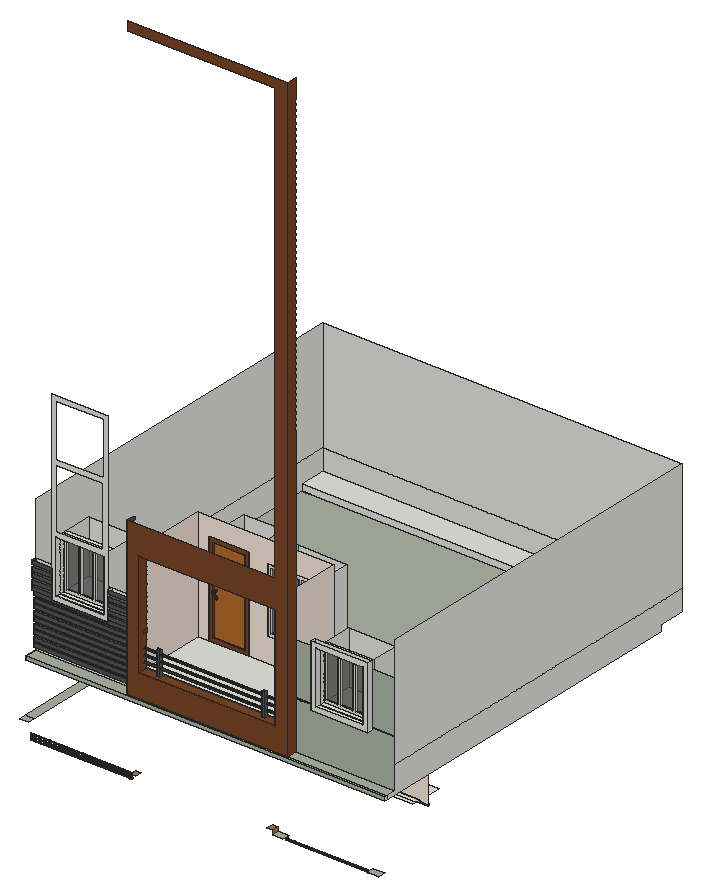
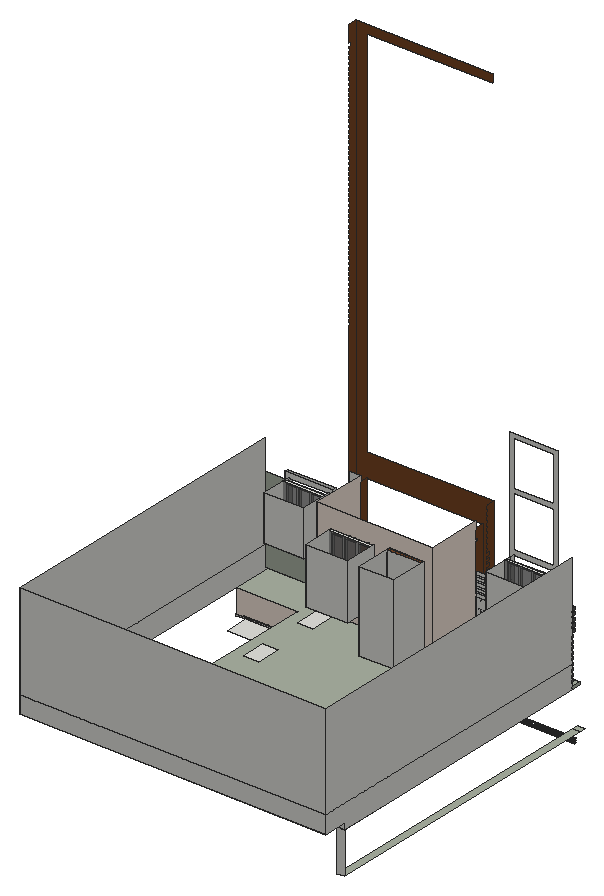
# SketchUp Ruby script. Lengths in inches.
U = 1.inch
M = Sketchup.active_model
def pt(a) = Geom::Point3d.new(a.map { |v| v * U })
def face(e, loops, mat)
  f = e.add_face(loops[0].map { |a| pt(a) })
  loops[1..].each { |l| e.add_face(l.map { |a| pt(a) }).erase! }
  f.material = f.back_material = mat if mat
  f
end
# faces: each face lists its corners as indices into pts; further lists are holes
def faces(e, pts, list, mat = nil) = list.each { |f| face(e, (f[0].is_a?(Array) ? f : [f]).map { |l| l.map { |i| pts[i] } }, mat) }
# xy, xz, yz: faces in a plane at the given z, y or x. An outline is a flat list of corners, or four numbers for a rectangle; further outlines are holes
def ring(l) = l.size == 4 ? [[l[0], l[1]], [l[2], l[1]], [l[2], l[3]], [l[0], l[3]]] : l.each_slice(2).to_a
def flat(e, list, mat, &to3) = list.each { |f| face(e, (f[0].is_a?(Array) ? f : [f]).map { |l| ring(l).map { |u, v| to3.(u, v) } }, mat) }
def xy(e, z, list, mat = nil) = flat(e, list, mat) { |x, y| [x, y, z] }
def xz(e, y, list, mat = nil) = flat(e, list, mat) { |x, z| [x, y, z] }
def yz(e, x, list, mat = nil) = flat(e, list, mat) { |y, z| [x, y, z] }
def lines(e, pts, list) = list.each { |a, b| e.add_line(pt(pts[a]), pt(pts[b])) }
# prism: a flat outline (further loops are holes) pulled along v
def prism(e, loops, v, mat = nil)
  f = face(e, loops, mat); d = Geom::Vector3d.new(v.map { |x| x * U })
  f.pushpull(f.normal.samedirection?(d) ? d.length : -d.length)
end
def box(e, o, s, mat = nil) = prism(e, [[o, [o[0] + s[0], o[1], o[2]], [o[0] + s[0], o[1] + s[1], o[2]], [o[0], o[1] + s[1], o[2]]]], [0, 0, s[2]], mat)
def at(x, y, z, deg = 0) = Geom::Transformation.translation(pt([x, y, z])) * Geom::Transformation.rotation(ORIGIN, Z_AXIS, deg.degrees)
def axes(o, x, y, z) = Geom::Transformation.new([*x, 0, *y, 0, *z, 0, *pt(o).to_a, 1])
def part(name) = M.definitions.add(name)
# library, detail: a bought-in or finely detailed component or shape, given as its bounding box
def library(name, o, s) = part(name).tap { |d| box(d.entities, o, s) }
def detail(e, o, s) = box(e.add_group.entities, o, s)
def put(e, d, t, mat = nil) = e.add_instance(d, t).tap { |i| i.material = mat if mat }
def group(e, t, mat = nil) = e.add_group.tap { |g| g.transformation = t; g.material = mat if mat }.entities
root = M.entities
M.materials.add("Generic\#1").color = [85, 85, 85]
M.materials.add("Generic\#2").color = [170, 178, 163]
M.materials.add("Generic\#3").color = [162, 123, 74]
M.materials.add("Generic\#4").color = [241, 227, 216]
M.materials.add("[Color M07]").color = [58, 58, 58]
M.materials.add("[Translucent Glass Gray]").color = [91, 91, 91]
M.materials["[Translucent Glass Gray]"].alpha = 0.55
M.materials.add("[Wood Bamboo]").color = [177, 105, 43]
M.materials.add("[Wood Veneer 01]").color = [120, 70, 37]
c1 = part("Group\#4")
xy(c1.entities,0,[[0,0,168,3.625]])
xy(c1.entities,5.375,[[0,0,168,3.625]])
xz(c1.entities,0,[[0,0,168,5.375]])
yz(c1.entities,0,[[0,0,3.625,5.375]])
c2 = part("Group\#3")
xy(c2.entities,0,[[0,4.93,60.125,10.18]])
xy(c2.entities,5.66,[[5.66,4.93,54.46,7.18]],"[Wood Veneer 01]")
xy(c2.entities,68.44,[[8.18,1.47,8.18,7.18,9.93,7.18,9.93,2.62]],"[Color M07]")
xy(c2.entities,70.41,[[8.19,0,9.94,1.15,9.94,7.18,8.19,7.18]],"[Color M07]")
xy(c2.entities,134.78,[[5.66,4.93,54.46,7.18]])
xy(c2.entities,140.4375,[[0,4.93,60.125,10.18]],"[Wood Veneer 01]")
xz(c2.entities,4.93,[[[0,0,60.125,140.4375],[5.66,5.66,54.46,134.78]]],"[Wood Veneer 01]")
xz(c2.entities,7.18,[[[5.66,5.66,54.46,134.78],[8.18,68.44,8.19,70.41,9.94,70.41,9.93,68.44]],[8.18,68.44,8.19,70.41,9.94,70.41,9.93,68.44]],"[Wood Bamboo]")
xz(c2.entities,10.18,[[0,0,60.125,140.4375]])
yz(c2.entities,0,[[4.93,0,10.18,140.4375]],"[Wood Veneer 01]")
yz(c2.entities,5.66,[[4.93,5.66,7.18,134.78]],"[Wood Veneer 01]")
yz(c2.entities,54.46,[[4.93,5.66,7.18,134.78]],"[Wood Veneer 01]")
yz(c2.entities,60.125,[[4.93,0,10.18,140.4375]],"[Wood Veneer 01]")
p = [[8.19,0,70.41],[8.18,1.47,68.44],[14.45,1.47,61.21],[15.43,0,62.06],[15.45,2.62,62.07],[16.43,1.15,62.92],
  [9.93,2.62,68.44],[9.94,1.15,70.41],[8.19,7.18,70.41],[8.18,7.18,68.44],[9.93,7.18,68.44],[9.94,7.18,70.41],
  [8.95,0.93,69.83],[15.58,0.93,62.1875],[8.95,7.18,69.83]]
faces(c2.entities,p,[[0,1,2,3],[3,2,4,5],[1,6,4,2],[7,0,3,5],[6,7,5,4],[8,9,1,0],[10,11,7,6]],"[Color M07]")
lines(c2.entities,p,[[12,13],[14,12]])
c3 = part("Group\#2")
xy(c3.entities,0,[[0,0,74.5625,5.5]])
xy(c3.entities,4.83,[[4.83,0,23.24,2.5],[28.07,0,46.49,2.5],[51.32,0,69.73,2.5]])
xy(c3.entities,93.17,[[4.83,0,23.24,2.5],[28.07,0,46.49,2.5],[51.32,0,69.73,2.5]])
xy(c3.entities,98,[[0,0,74.5625,5.5]])
xz(c3.entities,0,[[[0,0,74.5625,98],[28.07,4.83,46.49,93.17],[51.32,4.83,69.73,93.17],[4.83,4.83,23.24,93.17]]])
xz(c3.entities,2.5,[[4.83,4.83,23.24,93.17],[28.07,4.83,46.49,93.17],[51.32,4.83,69.73,93.17]],"[Translucent Glass Gray]")
xz(c3.entities,5.5,[[0,0,74.5625,98]],"[Translucent Glass Gray]")
yz(c3.entities,0,[[0,0,5.5,98]])
yz(c3.entities,4.83,[[0,4.83,2.5,93.17]])
yz(c3.entities,23.24,[[0,4.83,2.5,93.17]])
yz(c3.entities,28.07,[[0,4.83,2.5,93.17]])
yz(c3.entities,46.49,[[0,4.83,2.5,93.17]])
yz(c3.entities,51.32,[[0,4.83,2.5,93.17]])
yz(c3.entities,69.73,[[0,4.83,2.5,93.17]])
yz(c3.entities,74.5625,[[0,0,5.5,98]])
c4 = part("Group\#1")
xy(c4.entities,0,[[0,0,70.8125,6.0625]])
xy(c4.entities,4.26,[[4.26,0,22.19,2.0625],[26.44,0,44.37,2.0625],[48.63,0,66.56,2.0625]])
xy(c4.entities,75.06,[[4.26,0,22.19,2.0625],[26.44,0,44.37,2.0625],[48.63,0,66.56,2.0625]])
xy(c4.entities,79.3125,[[0,0,70.8125,6.0625]])
xz(c4.entities,0,[[[0,0,70.8125,79.3125],[26.44,4.26,44.37,75.06],[4.26,4.26,22.19,75.06],[48.63,4.26,66.56,75.06]]])
xz(c4.entities,2.0625,[[4.26,4.26,22.19,75.06],[26.44,4.26,44.37,75.06],[48.63,4.26,66.56,75.06]],"[Translucent Glass Gray]")
xz(c4.entities,6.0625,[[0,0,70.8125,79.3125]],"[Translucent Glass Gray]")
yz(c4.entities,0,[[0,0,6.0625,79.3125]])
yz(c4.entities,4.26,[[0,4.26,2.0625,75.06]])
yz(c4.entities,22.19,[[0,4.26,2.0625,75.06]])
yz(c4.entities,26.44,[[0,4.26,2.0625,75.06]])
yz(c4.entities,44.37,[[0,4.26,2.0625,75.06]])
yz(c4.entities,48.63,[[0,4.26,2.0625,75.06]])
yz(c4.entities,66.56,[[0,4.26,2.0625,75.06]])
yz(c4.entities,70.8125,[[0,0,6.0625,79.3125]])
xy(root,58.9,[[16.75,5.31,169.3125,6.62]],"Generic\#1")
xy(root,59.38,[[410.9,5.97,412.55,5.97,412.7,6.16,412.8125,6.43,412.85,6.72,412.8125,7.02,412.7,7.29,412.55,7.48,410.9,7.48,410.75,7.29,410.64,7.02,410.6,6.72,410.64,6.43,410.75,6.16],[512.09,5.97,513.74,5.97,513.89,6.16,514,6.43,514.04,6.72,514,7.02,513.89,7.29,513.74,7.48,512.09,7.48,511.94,7.29,511.83,7.02,511.79,6.72,511.83,6.43,511.94,6.16]])
xy(root,59.38,[[411.73,5.6,412.02,5.64,412.29,5.75,412.52,5.93,412.55,5.97,410.9,5.97,410.93,5.93,411.17,5.75,411.4375,5.64],[512.92,5.6,513.21,5.64,513.48,5.75,513.71,5.93,513.74,5.97,512.09,5.97,512.12,5.93,512.35,5.75,512.625,5.64],[410.9,7.48,412.55,7.48,412.52,7.52,412.29,7.7,412.02,7.8125,411.73,7.85,411.4375,7.8125,411.17,7.7,410.93,7.52],[512.09,7.48,513.74,7.48,513.71,7.52,513.48,7.7,513.21,7.8125,512.92,7.85,512.625,7.8125,512.35,7.7,512.12,7.52]],"Generic\#1")
xy(root,59.84,[[16.75,5.31,169.3125,6.62]],"Generic\#1")
xy(root,61.1875,[[383.68,1.625,399.68,12.1875],[526.51,1.625,543.6875,12.1875]],"Generic\#2")
xy(root,62.53,[[16.75,5.31,169.3125,6.62]],"Generic\#1")
xy(root,63.47,[[16.75,5.31,169.3125,6.62]],"Generic\#1")
xy(root,66.15,[[16.75,5.31,169.3125,6.62]],"Generic\#1")
xy(root,67.09,[[16.75,5.31,169.3125,6.62]],"Generic\#1")
xy(root,67.4375,[[43.38,5.24,44.57,6.49],[92.71,5.24,93.9,6.49],[142.04,5.24,143.23,6.49]],"Generic\#1")
xy(root,67.5625,[[169.3125,1.625,177.3125,12.1875],[375.68,1.625,383.68,12.1875]],"Generic\#3")
xy(root,84.25,[[3.6875,1.625,16.75,12.1875],[3.6875,12.1875,16.75,531.1875]],"Generic\#2")
xy(root,114.9375,[[455.38,87.75,526.46,94.125],[455.38,94.125,526.46,135.5]])
xy(root,115.46,[[435.75,94.125,451.03,95.75],[530.8125,94.125,543.6875,95.75]])
xy(root,117.46,[[435.75,94.125,451.03,95.75],[530.8125,94.125,543.6875,95.75]])
xy(root,119.29,[[451.03,87.75,530.8125,94.125]])
xy(root,158.4375,[[3.6875,12.1875,543.6875,15.8125],[3.6875,15.8125,3.6875,531.1875,435.75,531.1875,435.75,94.125,543.6875,94.125,543.6875,15.8125]],"Generic\#2")
xy(root,163.8125,[[153.3125,15.8125,395.4375,31.0625],[142.43,83.81,169.24,125.75],[383.68,83.81,410.49,125.75],[142.43,202,169.24,243.94],[383.68,202,410.49,243.94],
  [142.43,320.19,169.24,362.12],[383.68,320.19,410.49,320.19,410.49,362.12,383.68,362.12,383.68,361.87,405.71,361.87,405.71,322.81,383.68,322.81],[380.34,322.81,383.68,361.87],[383.68,322.81,405.71,361.87]])
xy(root,163.8125,[[3.6875,12.1875,543.6875,12.1875,543.6875,15.8125,153.3125,15.8125,153.3125,31.0625,3.6875,31.0625],[395.4375,15.8125,543.6875,31.0625]],"Generic\#2")
xy(root,168,[[3.6875,531.1875,543.6875,571.0625]])
xy(root,198.875,[[351.19,22.73,355.76,26.42],[171.6875,31.0625,171.6875,127,187.38,127,187.38,193.75,247.51,193.75,247.51,127,375.6875,127,375.6875,31.0625]])
xy(root,198.875,[[[171.6875,15.8125,375.6875,31.0625],[351.19,22.73,355.76,26.42],[192.01,22.73,196.57,26.42]]],"[Wood Veneer 01]")
xy(root,209.02,[[171.6875,23.99,375.6875,25.8]],"Generic\#1")
xy(root,210.64,[[171.6875,23.99,375.6875,25.8]],"Generic\#1")
xy(root,218.27,[[171.6875,23.99,375.6875,25.8]],"Generic\#1")
xy(root,219.89,[[171.6875,23.99,375.6875,25.8]],"Generic\#1")
xy(root,227.52,[[171.6875,23.99,375.6875,25.8]],"Generic\#1")
xy(root,229.14,[[171.6875,23.99,375.6875,25.8]],"Generic\#1")
xy(root,233.03,[[423.8125,24.0625,508.98,31.0625]])
xy(root,234.1875,[[192.01,22.73,196.57,26.42],[351.19,22.73,355.76,26.42]],"Generic\#1")
xy(root,235.875,[[395.4375,31.0625,423.8125,32.9375],[508.98,31.0625,543.6875,32.9375]])
xy(root,235.91,[[275.98,127,350.54,183.625]])
xy(root,237.875,[[395.4375,31.0625,423.8125,32.9375],[508.98,31.0625,543.6875,32.9375]])
xy(root,240.2,[[430.99,24.0625,501.8,31.0625],[430.99,31.0625,501.8,85.4375]])
xy(root,245.21,[[33.1875,24.0625,118.35,31.0625]],"Generic\#1")
xy(root,247.625,[[3.6875,24.0625,33.1875,31.0625],[118.35,24.0625,153.3125,31.0625]],"Generic\#1")
xy(root,252.39,[[40.36,24.0625,111.18,31.0625],[40.36,31.0625,111.18,85.4375]])
xy(root,253,[[3.6875,24.0625,33.1875,31.0625],[118.35,24.0625,153.3125,31.0625]],"Generic\#1")
xy(root,256.3125,[[3.6875,24.0625,33.1875,31.0625],[118.35,24.0625,153.3125,31.0625]],"Generic\#1")
xy(root,261.6875,[[3.6875,24.0625,33.1875,31.0625],[118.35,24.0625,153.3125,31.0625]],"Generic\#1")
xy(root,265,[[3.6875,24.0625,33.1875,31.0625],[118.35,24.0625,153.3125,31.0625]],"Generic\#1")
xy(root,270.375,[[3.6875,24.0625,33.1875,31.0625],[118.35,24.0625,153.3125,31.0625]],"Generic\#1")
xy(root,273.6875,[[3.6875,24.0625,33.1875,31.0625],[118.35,24.0625,153.3125,31.0625]],"Generic\#1")
xy(root,279.0625,[[118.35,31.0625,153.3125,35.3125]])
xy(root,279.0625,[[3.6875,24.0625,33.1875,31.0625],[118.35,24.0625,153.3125,31.0625]],"Generic\#1")
xy(root,282.375,[[118.35,31.0625,153.3125,35.3125]])
xy(root,282.375,[[3.6875,24.0625,33.1875,31.0625],[118.35,24.0625,153.3125,31.0625]],"Generic\#1")
xz(root,5.31,[[16.75,58.9,169.3125,59.84],[16.75,62.53,169.3125,63.47],[16.75,66.15,169.3125,67.09]],"Generic\#1")
xz(root,6.62,[[16.75,58.9,169.3125,59.84],[16.75,62.53,169.3125,63.47],[16.75,66.15,169.3125,67.09]])
xz(root,12.1875,[[3.6875,158.4375,543.6875,163.8125]],"Generic\#2")
xz(root,15.8125,[[[153.3125,163.8125,395.4375,163.8125,395.4375,1071.875,154.5,1071.875,154.5,1058.1875,375.6875,1058.1875,375.6875,397.75,153.3125,397.75],[171.6875,198.875,375.6875,356.125]]],"[Wood Veneer 01]")
xz(root,22.73,[[192.01,198.875,196.57,234.1875],[351.19,198.875,355.76,234.1875]],"Generic\#1")
xz(root,23.99,[[171.6875,209.02,375.6875,210.64],[171.6875,218.27,375.6875,219.89],[171.6875,227.52,375.6875,229.14]],"Generic\#1")
xz(root,24.0625,[[[423.8125,233.03,508.98,326.69],[430.99,240.2,501.8,319.52]],[[33.1875,245.21,118.35,522.69],[40.375,338.88,110.67,429.03],[40.36,252.39,111.18,331.7],[40.36,436.2,111.18,515.52]]])
xz(root,24.0625,[[3.6875,247.625,33.1875,253],[118.35,247.625,153.3125,253],[153.3125,247.625,171.6875,253],[40.36,252.39,111.18,253],[3.6875,256.3125,33.1875,261.6875],
  [118.35,256.3125,153.3125,261.6875],[3.6875,265,33.1875,270.375],[118.35,265,153.3125,270.375],[3.6875,273.6875,33.1875,279.0625],[118.35,273.6875,153.3125,279.0625],
  [3.6875,282.375,33.1875,287.75],[118.35,282.375,153.3125,287.75]],"Generic\#1")
xz(root,25.8,[[171.6875,209.02,375.6875,210.64],[171.6875,218.27,375.6875,219.89],[171.6875,227.52,375.6875,229.14]])
xz(root,26.42,[[192.01,198.875,196.57,234.1875],[351.19,198.875,355.76,234.1875]])
xz(root,31.0625,[[3.6875,163.8125,153.3125,163.8125,153.3125,247.625,118.35,247.625,118.35,245.21,33.1875,245.21,33.1875,247.625,3.6875,247.625],[153.3125,163.8125,395.4375,198.875],[153.3125,198.875,171.6875,247.625],[375.6875,198.875,395.4375,366.875],[[423.8125,233.03,508.98,326.69],[430.99,240.2,501.8,319.52]],
  [33.1875,245.21,118.35,247.625],[3.6875,247.625,33.1875,253],[33.1875,247.625,33.1875,253,40.36,253,40.36,252.39,111.18,252.39,111.18,253,118.35,253,118.35,247.625],[118.35,247.625,153.3125,253],[153.3125,247.625,171.6875,253],
  [3.6875,253,33.1875,256.3125],[33.1875,253,40.36,256.3125],[111.18,253,118.35,256.3125],[118.35,253,153.3125,256.3125],[153.3125,253,171.6875,256.3125],
  [3.6875,256.3125,33.1875,261.6875],[33.1875,256.3125,40.36,261.6875],[111.18,256.3125,118.35,261.6875],[118.35,256.3125,153.3125,261.6875],[153.3125,256.3125,171.6875,261.6875],
  [3.6875,261.6875,33.1875,265],[33.1875,261.6875,40.36,265],[111.18,261.6875,118.35,265],[118.35,261.6875,153.3125,265],[153.3125,261.6875,171.6875,265],
  [3.6875,265,33.1875,270.375],[33.1875,265,40.36,270.375],[111.18,265,118.35,270.375],[118.35,265,153.3125,270.375],[153.3125,265,171.6875,270.375],
  [3.6875,270.375,33.1875,273.6875],[33.1875,270.375,40.36,273.6875],[111.18,270.375,118.35,273.6875],[118.35,270.375,153.3125,273.6875],[153.3125,270.375,171.6875,273.6875],
  [3.6875,273.6875,33.1875,279.0625],[33.1875,273.6875,40.36,279.0625],[111.18,273.6875,118.35,279.0625],[118.35,273.6875,153.3125,279.0625],[153.3125,273.6875,171.6875,279.0625],
  [3.6875,279.0625,33.1875,282.375],[33.1875,279.0625,40.36,282.375],[111.18,279.0625,118.35,282.375],[118.35,279.0625,153.3125,282.375],[153.3125,279.0625,171.6875,282.375],
  [3.6875,282.375,33.1875,287.75],[33.1875,282.375,40.36,287.75],[111.18,282.375,118.35,287.75],[118.35,282.375,153.3125,287.75],[153.3125,282.375,171.6875,287.75]])
xz(root,31.0625,[[395.4375,163.8125,543.6875,163.8125,543.6875,235.875,508.98,235.875,508.98,233.03,423.8125,233.03,423.8125,235.875,395.4375,235.875],[395.4375,237.875,423.8125,315.5],[508.98,237.875,543.6875,315.5]],"Generic\#2")
xz(root,32.9375,[[395.4375,235.875,423.8125,237.875],[508.98,235.875,543.6875,237.875]],"Generic\#1")
xz(root,35.3125,[[118.35,279.0625,153.3125,282.375]])
xz(root,85.4375,[[430.99,240.2,501.8,319.52],[40.36,252.39,111.18,331.7]])
xz(root,94.125,[[451.03,115.46,530.8125,117.46],[451.03,117.46,530.8125,119.29]])
xz(root,94.125,[[435.75,117.46,451.03,117.46,451.03,119.29,530.8125,119.29,530.8125,117.46,543.6875,117.46,543.6875,158.4375,435.75,158.4375]],"Generic\#4")
xz(root,95.75,[[435.75,115.46,451.03,117.46],[530.8125,115.46,543.6875,117.46]])
xz(root,127,[[[171.6875,198.875,187.38,198.875,187.38,339.3125,247.51,339.3125,247.51,198.875,375.6875,198.875,375.6875,366.875,171.6875,366.875],[275.98,235.91,350.54,333.91]]],"Generic\#4")
xz(root,183.625,[[275.98,235.91,350.54,333.91]])
xz(root,193.75,[[187.38,198.875,247.51,339.3125]])
xz(root,531.1875,[[3.6875,84.25,16.75,158.4375],[3.6875,158.4375,543.6875,168]])
xz(root,571.0625,[[3.6875,168,543.6875,198.875],[3.6875,198.875,543.6875,366.875]])
yz(root,3.6875,[[31.0625,158.4375,31.0625,198.875,571.0625,198.875,571.0625,168,531.1875,168,531.1875,158.4375],[31.0625,198.875,571.0625,366.875]])
yz(root,3.6875,[[24.0625,247.625,31.0625,253],[24.0625,256.3125,31.0625,261.6875],[24.0625,265,31.0625,270.375],[24.0625,273.6875,31.0625,279.0625],[24.0625,282.375,31.0625,287.75]],"Generic\#1")
yz(root,3.6875,[[12.1875,158.4375,31.0625,163.8125]],"Generic\#2")
yz(root,16.75,[[5.31,58.9,6.62,59.84],[5.31,62.53,6.62,63.47],[5.31,66.15,6.62,67.09]],"Generic\#2")
yz(root,33.1875,[[24.0625,245.21,31.0625,247.625],[24.0625,247.625,31.0625,253],[24.0625,253,31.0625,256.3125],[24.0625,256.3125,31.0625,261.6875],[24.0625,261.6875,31.0625,265],
  [24.0625,265,31.0625,270.375],[24.0625,270.375,31.0625,273.6875],[24.0625,273.6875,31.0625,279.0625],[24.0625,279.0625,31.0625,282.375],[24.0625,282.375,31.0625,287.75]])
yz(root,40.36,[[24.0625,252.39,31.0625,331.7],[31.0625,252.39,85.4375,331.7]])
yz(root,111.18,[[24.0625,252.39,31.0625,331.7],[31.0625,252.39,85.4375,331.7]])
yz(root,118.35,[[24.0625,245.21,31.0625,247.625],[24.0625,247.625,31.0625,253],[24.0625,253,31.0625,256.3125],[24.0625,256.3125,31.0625,261.6875],[24.0625,261.6875,31.0625,265],
  [24.0625,265,31.0625,270.375],[24.0625,270.375,31.0625,273.6875],[24.0625,273.6875,31.0625,279.0625],[24.0625,279.0625,31.0625,282.375],[31.0625,279.0625,35.3125,282.375],
  [24.0625,282.375,31.0625,287.75]])
yz(root,153.3125,[[24.0625,247.625,31.0625,253],[24.0625,256.3125,31.0625,261.6875],[24.0625,265,31.0625,270.375],[24.0625,273.6875,31.0625,279.0625],[31.0625,279.0625,35.3125,282.375],
  [24.0625,282.375,31.0625,287.75]])
yz(root,153.3125,[[15.8125,163.8125,15.8125,397.75,27.4375,397.75,27.4375,395.3125,31.0625,395.3125,31.0625,392,27.4375,392,27.4375,386.625,31.0625,386.625,31.0625,383.3125,27.4375,383.3125,27.4375,377.9375,31.0625,377.9375,31.0625,374.625,27.4375,374.625,27.4375,369.25,31.0625,369.25,31.0625,365.9375,27.4375,365.9375,27.4375,360.5625,31.0625,360.5625,31.0625,357.25,27.4375,357.25,27.4375,351.875,31.0625,351.875,31.0625,348.5625,27.4375,348.5625,27.4375,343.1875,31.0625,343.1875,31.0625,338.88,27.75,338.88,27.75,334.5,31.0625,334.5,31.0625,331.1875,27.75,331.1875,27.75,325.8125,31.0625,325.8125,31.0625,322.5,24.0625,322.5,24.0625,317.125,31.0625,317.125,31.0625,313.8125,24.0625,313.8125,24.0625,308.4375,31.0625,308.4375,31.0625,305.125,24.0625,305.125,24.0625,299.75,31.0625,299.75,31.0625,296.4375,24.0625,296.4375,24.0625,291.0625,31.0625,291.0625,31.0625,287.75,24.0625,287.75,24.0625,282.375,31.0625,282.375,31.0625,279.0625,24.0625,279.0625,24.0625,273.6875,31.0625,273.6875,31.0625,270.375,24.0625,270.375,24.0625,265,31.0625,265,31.0625,261.6875,24.0625,261.6875,24.0625,256.3125,31.0625,256.3125,31.0625,253,24.0625,253,24.0625,247.625,31.0625,247.625,31.0625,163.8125]],"[Wood Veneer 01]")
yz(root,169.3125,[[5.31,58.9,6.62,59.84],[5.31,62.53,6.62,63.47],[5.31,66.15,6.62,67.09]])
yz(root,171.6875,[[23.99,209.02,25.8,210.64],[23.99,218.27,25.8,219.89],[23.99,227.52,25.8,229.14]])
yz(root,171.6875,[[31.0625,198.875,127,366.875]],"Generic\#4")
yz(root,171.6875,[[[15.8125,198.875,31.0625,198.875,31.0625,247.625,24.0625,247.625,24.0625,253,31.0625,253,31.0625,334.5,27.75,334.5,27.75,338.88,31.0625,338.88,31.0625,356.125,15.8125,356.125],[23.99,227.52,25.8,229.14],[23.99,218.27,25.8,219.89],[23.99,209.02,25.8,210.64]],[24.0625,247.625,31.0625,253]],"[Wood Veneer 01]")
yz(root,187.38,[[127,198.875,193.75,339.3125]])
yz(root,192.01,[[22.73,198.875,26.42,234.1875]],"Generic\#1")
yz(root,196.57,[[22.73,198.875,26.42,234.1875]],"Generic\#1")
yz(root,247.51,[[127,198.875,193.75,339.3125]])
yz(root,275.98,[[127,235.91,183.625,333.91]])
yz(root,350.54,[[127,235.91,183.625,333.91]])
yz(root,351.19,[[22.73,198.875,26.42,234.1875]],"Generic\#1")
yz(root,355.76,[[22.73,198.875,26.42,234.1875]],"Generic\#1")
yz(root,375.6875,[[31.0625,198.875,127,366.875]],"Generic\#4")
yz(root,375.6875,[[[15.8125,198.875,31.0625,356.125],[23.99,209.02,25.8,210.64],[23.99,218.27,25.8,219.89],[23.99,227.52,25.8,229.14]]],"[Wood Veneer 01]")
yz(root,383.68,[[1.625,61.1875,12.1875,67.5625]],"Generic\#3")
yz(root,395.4375,[[31.0625,235.875,32.9375,237.875]])
yz(root,395.4375,[[15.8125,163.8125,31.0625,163.8125,31.0625,596.625,28.5,596.625,28.5,602.125,31.0625,602.125,31.0625,604.9375,28.5,604.9375,28.5,610.4375,31.0625,610.4375,31.0625,613.25,28.5,613.25,28.5,618.75,31.0625,618.75,31.0625,621.5625,28.5,621.5625,28.5,627.0625,31.0625,627.0625,31.0625,629.875,28.5,629.875,28.5,635.375,31.0625,635.375,31.0625,638.1875,28.5,638.1875,28.5,643.6875,31.0625,643.6875,31.0625,646.5,28.5,646.5,28.5,652,31.0625,652,31.0625,654.8125,28.5,654.8125,28.5,660.3125,31.0625,660.3125,31.0625,663.125,28.5,663.125,28.5,668.625,31.0625,668.625,31.0625,671.4375,28.5,671.4375,28.5,676.9375,31.0625,676.9375,31.0625,679.75,28.5,679.75,28.5,685.25,31.0625,685.25,31.0625,688.0625,28.5,688.0625,28.5,693.5625,31.0625,693.5625,31.0625,696.375,28.5,696.375,28.5,701.875,31.0625,701.875,31.0625,704.6875,28.5,704.6875,28.5,710.1875,31.0625,710.1875,31.0625,713,28.5,713,28.5,718.5,31.0625,718.5,31.0625,721.3125,28.5,721.3125,28.5,726.8125,31.0625,726.8125,31.0625,729.625,28.5,729.625,28.5,735.125,31.0625,735.125,31.0625,737.9375,28.5,737.9375,28.5,743.4375,31.0625,743.4375,31.0625,746.25,28.5,746.25,28.5,751.75,31.0625,751.75,31.0625,754.5625,28.5,754.5625,28.5,760.0625,31.0625,760.0625,31.0625,762.875,28.5,762.875,28.5,768.375,31.0625,768.375,31.0625,771.1875,28.5,771.1875,28.5,776.6875,31.0625,776.6875,31.0625,779.5,28.5,779.5,28.5,785,31.0625,785,31.0625,787.8125,28.5,787.8125,28.5,793.3125,31.0625,793.3125,31.0625,796.125,28.5,796.125,28.5,801.625,31.0625,801.625,31.0625,804.4375,28.5,804.4375,28.5,809.9375,31.0625,809.9375,31.0625,812.75,28.5,812.75,28.5,818.25,31.0625,818.25,31.0625,821.0625,28.5,821.0625,28.5,826.5625,31.0625,826.5625,31.0625,829.375,28.5,829.375,28.5,834.875,31.0625,834.875,31.0625,837.6875,28.5,837.6875,28.5,843.1875,31.0625,843.1875,31.0625,846,28.5,846,28.5,851.5,31.0625,851.5,31.0625,854.3125,28.5,854.3125,28.5,859.8125,31.0625,859.8125,31.0625,862.625,28.5,862.625,28.5,868.125,31.0625,868.125,31.0625,870.9375,28.5,870.9375,28.5,876.4375,31.0625,876.4375,31.0625,879.25,28.5,879.25,28.5,884.75,31.0625,884.75,31.0625,887.5625,28.5,887.5625,28.5,893.0625,31.0625,893.0625,31.0625,895.875,28.5,895.875,28.5,901.375,31.0625,901.375,31.0625,904.1875,28.5,904.1875,28.5,909.6875,31.0625,909.6875,31.0625,912.5,28.5,912.5,28.5,918,31.0625,918,31.0625,920.8125,28.5,920.8125,28.5,926.3125,31.0625,926.3125,31.0625,929.125,28.5,929.125,28.5,934.625,31.0625,934.625,31.0625,937.4375,28.5,937.4375,28.5,942.9375,31.0625,942.9375,31.0625,945.75,28.5,945.75,28.5,951.25,31.0625,951.25,31.0625,954.0625,28.5,954.0625,28.5,959.5625,31.0625,959.5625,31.0625,962.375,28.5,962.375,28.5,967.875,31.0625,967.875,31.0625,970.6875,28.5,970.6875,28.5,976.1875,31.0625,976.1875,31.0625,979,28.5,979,28.5,984.5,31.0625,984.5,31.0625,987.3125,28.5,987.3125,28.5,992.8125,31.0625,992.8125,31.0625,995.625,28.5,995.625,28.5,1001.125,31.0625,1001.125,31.0625,1003.9375,28.5,1003.9375,28.5,1009.4375,31.0625,1009.4375,31.0625,1012.25,28.5,1012.25,28.5,1017.75,31.0625,1017.75,31.0625,1020.5625,28.5,1020.5625,28.5,1026.0625,31.0625,1026.0625,31.0625,1028.875,28.5,1028.875,28.5,1034.375,31.0625,1034.375,31.0625,1037.1875,28.1875,1037.1875,28.1875,1042.6875,31.0625,1042.6875,31.0625,1071.875,15.8125,1071.875]],"[Wood Veneer 01]")
yz(root,399.68,[[6.72,58.07,6.5,58.1,6.29,58.18,6.11,58.32,5.97,58.5,5.88,58.71,5.85,58.94,5.88,59.17,5.97,59.38,6.11,59.56,6.29,59.7,6.5,59.79,6.72,59.82,6.95,59.79,7.16,59.7,7.34,59.56,7.48,59.38,7.57,59.17,7.6,58.94,7.57,58.71,7.48,58.5,7.34,58.32,7.16,58.18,6.95,58.1]])
yz(root,423.8125,[[24.0625,233.03,31.0625,326.69],[31.0625,235.875,32.9375,237.875]])
yz(root,430.99,[[24.0625,240.2,31.0625,319.52],[31.0625,240.2,85.4375,319.52]])
yz(root,451.03,[[94.125,115.46,95.75,117.46]])
yz(root,501.8,[[24.0625,240.2,31.0625,319.52],[31.0625,240.2,85.4375,319.52]])
yz(root,508.98,[[24.0625,233.03,31.0625,326.69],[31.0625,235.875,32.9375,237.875]])
yz(root,530.8125,[[94.125,115.46,95.75,117.46]])
yz(root,543.6875,[[12.1875,158.4375,15.8125,163.8125],[15.8125,158.4375,531.1875,158.4375,531.1875,168,571.0625,168,571.0625,198.875,31.0625,198.875,31.0625,163.8125,15.8125,163.8125],[31.0625,198.875,571.0625,198.875,571.0625,366.875,31.0625,366.875,31.0625,317.5,32.9375,317.5,32.9375,315.5,31.0625,315.5,31.0625,237.875,32.9375,237.875,32.9375,235.875,31.0625,235.875]])
p = [[399.68,6.29,58.18],[399.68,6.5,58.1],[526.51,6.5,58.1],[526.51,6.29,58.18],[399.68,6.72,58.07],[410.6,6.72,58.07],
  [411.73,6.72,58.07],[412.85,6.72,58.07],[511.79,6.72,58.07],[512.92,6.72,58.07],[514.04,6.72,58.07],[526.51,6.72,58.07],
  [399.68,6.95,58.1],[526.51,6.95,58.1],[399.68,7.16,58.18],[526.51,7.16,58.18],[399.68,6.11,58.32],[526.51,6.11,58.32],
  [399.68,7.34,58.32],[526.51,7.34,58.32],[399.68,5.97,58.5],[526.51,5.97,58.5],[399.68,7.48,58.5],[526.51,7.48,58.5],
  [399.68,5.88,58.71],[526.51,5.88,58.71],[399.68,7.57,58.71],[526.51,7.57,58.71],[399.68,5.85,58.94],[526.51,5.85,58.94],
  [399.68,7.6,58.94],[526.51,7.6,58.94],[399.68,5.88,59.17],[526.51,5.88,59.17],[399.68,7.57,59.17],[526.51,7.57,59.17],
  [399.68,5.97,59.38],[526.51,5.97,59.38],[513.74,5.97,59.38],[512.09,5.97,59.38],[412.55,5.97,59.38],[410.9,5.97,59.38],
  [399.68,7.48,59.38],[410.9,7.48,59.38],[412.55,7.48,59.38],[512.09,7.48,59.38],[513.74,7.48,59.38],[526.51,7.48,59.38],
  [399.68,6.11,59.56],[526.51,6.11,59.56],[399.68,7.34,59.56],[526.51,7.34,59.56],[399.68,6.29,59.7],[526.51,6.29,59.7],
  [399.68,7.16,59.7],[526.51,7.16,59.7],[399.68,6.5,59.79],[526.51,6.5,59.79],[399.68,6.95,59.79],[526.51,6.95,59.79],
  [399.68,6.72,59.82],[526.51,6.72,59.82],[171.6875,24.8,209.99],[375.6875,24.8,209.99],[171.6875,24.8,219.11],[375.6875,24.8,219.11],
  [171.6875,24.8,228.24],[194.87,24.8,228.24],[352.49,24.8,228.24],[195.08,24.125,198.875],[352.71,24.125,198.875],[375.6875,24.8,228.24],
  [40.36,31.0625,253],[111.18,31.0625,253],[399.68,6.72,58.94],[410.6,6.72,58.94],[512.92,6.72,58.94],[514.04,6.72,58.94],
  [411.73,6.72,58.94],[412.85,6.72,58.94],[526.51,6.72,58.94],[511.79,6.72,58.94],[169.3125,5.77,59.46],[142.52,5.77,59.46],
  [169.3125,5.77,63.08],[142.52,5.77,63.08],[169.3125,5.77,66.71],[142.52,5.77,66.71],[93.26,5.77,66.71],[93.26,5.77,59.46],
  [93.26,5.77,63.08],[43.99,5.77,66.71],[43.99,5.77,59.46],[43.99,5.77,63.08],[16.3125,5.77,66.71],[16.3125,5.77,59.46],
  [16.3125,5.77,63.08]]
faces(root,p,[[0,1,2,3],[1,4,5,6,7,8,9,10,11,2],[4,12,13,11,10,9,8,7,6,5],[12,14,15,13],[16,0,3,17],[14,18,19,15],[20,16,17,21],[18,22,23,19],
  [24,20,21,25],[22,26,27,23],[28,24,25,29],[26,30,31,27],[32,28,29,33],[30,34,35,31],[36,32,33,37,38,39,40,41],[34,42,43,44,45,46,47,35],
  [48,36,41,40,39,38,37,49],[42,50,51,47,46,45,44,43],[52,48,49,53],[50,54,55,51],[56,52,53,57],[54,58,59,55],[60,56,57,61],[58,60,61,59]],"Generic\#1")
lines(root,p,[[62,63],[64,65],[66,67],[67,68],[69,67],[70,68],[68,71],[72,73],[74,75],[76,77],[76,9],[78,6],
  [78,79],[77,80],[81,76],[75,78],[79,81],[82,83],[84,85],[86,87],[87,88],[87,85],[83,89],[85,90],
  [85,83],[90,89],[88,90],[88,91],[89,92],[90,93],[93,92],[91,93],[91,94],[92,95],[93,96]])
put(root,c1,at(3.6875,27.4375,169.4375),"Generic\#1")
put(root,c1,at(3.6875,27.4375,178.125),"Generic\#1")
put(root,c1,at(3.6875,27.4375,186.8125),"Generic\#1")
put(root,c1,at(3.6875,27.4375,195.5),"Generic\#1")
put(root,c2,at(187.38,122.07,198.875))
put(root,c1,at(3.6875,27.4375,204.1875),"Generic\#1")
put(root,c1,at(3.6875,27.4375,212.875),"Generic\#1")
put(root,c1,at(3.6875,27.4375,221.5625),"Generic\#1")
put(root,c1,at(3.6875,27.4375,230.25),"Generic\#1")
put(root,c3,at(275.98,127,235.91))
put(root,c1,at(3.6875,27.4375,238.9375),"Generic\#1")
put(root,c4,at(430.99,38.0625,240.2))
put(root,c4,at(40.36,38.0625,252.39))
